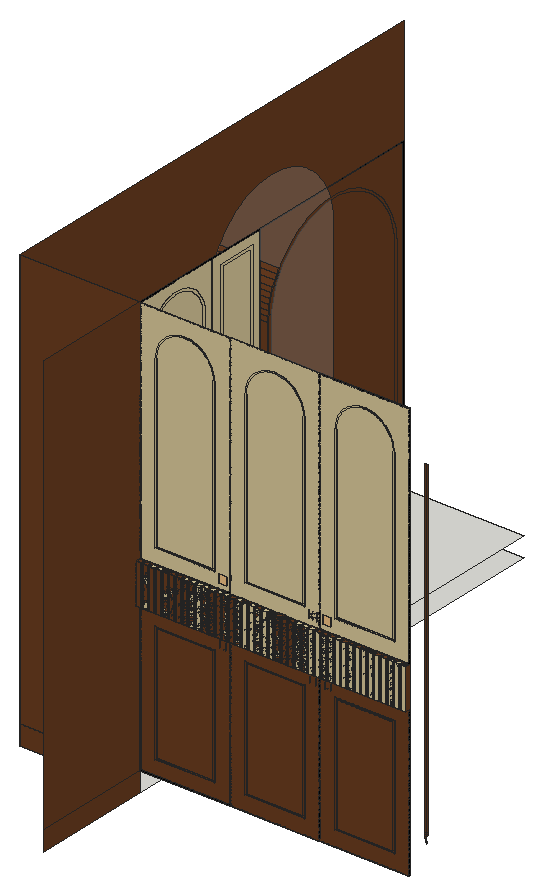
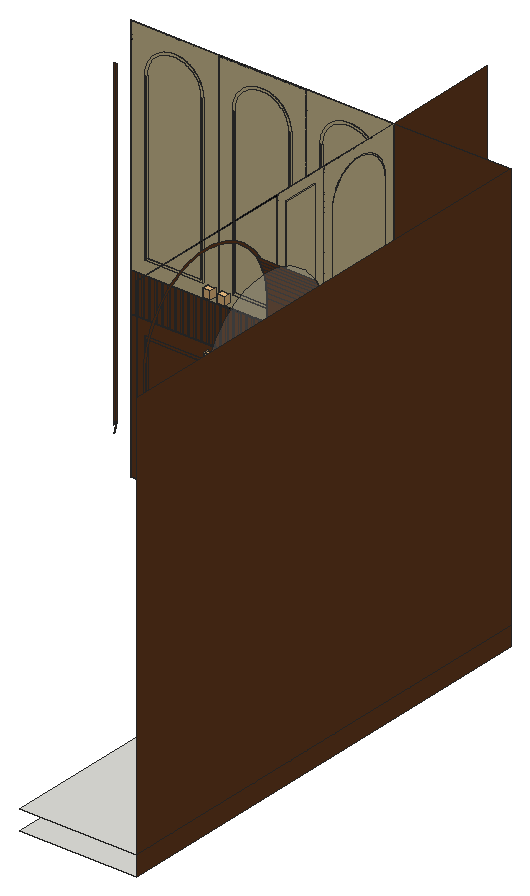
# SketchUp Ruby script. Lengths in inches.
U = 1.inch
M = Sketchup.active_model
def pt(a) = Geom::Point3d.new(a.map { |v| v * U })
def face(e, loops, mat)
  f = e.add_face(loops[0].map { |a| pt(a) })
  loops[1..].each { |l| e.add_face(l.map { |a| pt(a) }).erase! }
  f.material = f.back_material = mat if mat
  f
end
# faces: each face lists its corners as indices into pts; further lists are holes
def faces(e, pts, list, mat = nil) = list.each { |f| face(e, (f[0].is_a?(Array) ? f : [f]).map { |l| l.map { |i| pts[i] } }, mat) }
# xy, xz, yz: faces in a plane at the given z, y or x. An outline is a flat list of corners, or four numbers for a rectangle; further outlines are holes
def ring(l) = l.size == 4 ? [[l[0], l[1]], [l[2], l[1]], [l[2], l[3]], [l[0], l[3]]] : l.each_slice(2).to_a
def flat(e, list, mat, &to3) = list.each { |f| face(e, (f[0].is_a?(Array) ? f : [f]).map { |l| ring(l).map { |u, v| to3.(u, v) } }, mat) }
def xy(e, z, list, mat = nil) = flat(e, list, mat) { |x, y| [x, y, z] }
def xz(e, y, list, mat = nil) = flat(e, list, mat) { |x, z| [x, y, z] }
def yz(e, x, list, mat = nil) = flat(e, list, mat) { |y, z| [x, y, z] }
def lines(e, pts, list) = list.each { |a, b| e.add_line(pt(pts[a]), pt(pts[b])) }
# prism: a flat outline (further loops are holes) pulled along v
def prism(e, loops, v, mat = nil)
  f = face(e, loops, mat); d = Geom::Vector3d.new(v.map { |x| x * U })
  f.pushpull(f.normal.samedirection?(d) ? d.length : -d.length)
end
def box(e, o, s, mat = nil) = prism(e, [[o, [o[0] + s[0], o[1], o[2]], [o[0] + s[0], o[1] + s[1], o[2]], [o[0], o[1] + s[1], o[2]]]], [0, 0, s[2]], mat)
def at(x, y, z, deg = 0) = Geom::Transformation.translation(pt([x, y, z])) * Geom::Transformation.rotation(ORIGIN, Z_AXIS, deg.degrees)
def axes(o, x, y, z) = Geom::Transformation.new([*x, 0, *y, 0, *z, 0, *pt(o).to_a, 1])
def part(name) = M.definitions.add(name)
# library, detail: a bought-in or finely detailed component or shape, given as its bounding box
def library(name, o, s) = part(name).tap { |d| box(d.entities, o, s) }
def detail(e, o, s) = box(e.add_group.entities, o, s)
def put(e, d, t, mat = nil) = e.add_instance(d, t).tap { |i| i.material = mat if mat }
def group(e, t, mat = nil) = e.add_group.tap { |g| g.transformation = t; g.material = mat if mat }.entities
root = M.entities
M.materials.add("138_plaster painted wall texture-seamless").color = [214, 198, 153]
M.materials.add("[0137_Black]").color = [0, 0, 0]
M.materials.add("[Mirror 02]").color = [229, 229, 229]
M.materials["[Mirror 02]"].alpha = 0.23
M.materials.add("[Wood Veneer 01]").color = [104, 60, 32]
c1 = part("Group\#7")
box(c1.entities,[0,0,0],[1,1,8])
c2 = library("Group\#17",[0,0,0],[1.625,1.625,1.31])
xy(root,0,[[0,24,24,120]])
xy(root,4,[[0,24,24,120]])
xy(root,6,[[24,26,24.2,40],[24,44,24.2,52]],"[Wood Veneer 01]")
xy(root,6.4,[[24,26.4,24.2,39.6],[24,44.4,24.2,51.6]],"[Wood Veneer 01]")
xy(root,7,[[27,24,39,24.2]],"138_plaster painted wall texture-seamless")
xy(root,7,[[45,24,57,24.2],[63,24,75,24.2]],"[Wood Veneer 01]")
xy(root,7.4,[[27.4,24,38.6,24.2],[45.4,24,56.6,24.2],[63.4,24,74.6,24.2]],"[Wood Veneer 01]")
xy(root,30.6,[[27.4,24,38.6,24.2]],"138_plaster painted wall texture-seamless")
xy(root,30.6,[[45.4,24,56.6,24.2],[63.4,24,74.6,24.2]],"[Wood Veneer 01]")
xy(root,31,[[27,24,39,24.2],[45,24,57,24.2],[63,24,75,24.2]],"[Wood Veneer 01]")
xy(root,31.6,[[24,26.4,24.2,39.6]])
xy(root,31.6,[[24,44.4,24.2,51.6]],"[Wood Veneer 01]")
xy(root,32,[[24,26,24.2,40],[24,44,24.2,52]],"[Wood Veneer 01]")
xy(root,34,[[24,23,42,24],[42,23,60,24],[60,23,78,24]],"138_plaster painted wall texture-seamless")
xy(root,34,[[23,24,24,42],[23,42,24,54]],"[Wood Veneer 01]")
xy(root,36.4,[[12,56.4,24.2,87.6]],"[Wood Veneer 01]")
xy(root,42,[[24,23,42,24],[42,23,60,24],[60,23,78,24]],"138_plaster painted wall texture-seamless")
xy(root,42,[[23,24,24,42],[23,42,24,54]],"[Wood Veneer 01]")
xy(root,44,[[24,26,24.2,40],[24,44,24.2,52]])
xy(root,44.4,[[24,26.4,24.2,39.6],[24,44.4,24.2,51.6]])
xy(root,45,[[27,24,39,24.2],[45,24,57,24.2],[63,24,75,24.2]],"138_plaster painted wall texture-seamless")
xy(root,45.4,[[27.4,24,38.6,24.2],[45.4,24,56.6,24.2],[63.4,24,74.6,24.2]],"138_plaster painted wall texture-seamless")
xz(root,23,[[24,34,78,42]],"138_plaster painted wall texture-seamless")
xz(root,24,[[[24.1,42.1,41.9,87.9],[27,45,39,45,39,79,38.99,79.35,38.96,79.7,38.91,80.04,38.84,80.38,38.75,80.72,38.64,81.05,38.51,81.375,38.36,81.69,38.2,82,38.01,82.3,37.8125,82.58,37.6,82.86,37.36,83.12,37.12,83.36,36.86,83.6,36.58,83.8125,36.3,84.01,36,84.2,35.69,84.36,35.375,84.51,35.05,84.64,34.72,84.75,34.38,84.84,34.04,84.91,33.7,84.96,33.35,84.99,33,85,32.65,84.99,32.3,84.96,31.96,84.91,31.62,84.84,31.28,84.75,30.95,84.64,30.625,84.51,30.31,84.36,30,84.2,29.7,84.01,29.42,83.8125,29.14,83.6,28.88,83.36,28.64,83.12,28.4,82.86,28.1875,82.58,27.99,82.3,27.8,82,27.64,81.69,27.49,81.375,27.36,81.05,27.25,80.72,27.16,80.38,27.09,80.04,27.04,79.7,27.01,79.35,27,79]],[[42.1,42.1,59.9,87.9],[45,45,57,45,57,79,56.99,79.35,56.96,79.7,56.91,80.04,56.84,80.38,56.75,80.72,56.64,81.05,56.51,81.375,56.36,81.69,56.2,82,56.01,82.3,55.8125,82.58,55.6,82.86,55.36,83.12,55.12,83.36,54.86,83.6,54.58,83.8125,54.3,84.01,54,84.2,53.69,84.36,53.375,84.51,53.05,84.64,52.72,84.75,52.38,84.84,52.04,84.91,51.7,84.96,51.35,84.99,51,85,50.65,84.99,50.3,84.96,49.96,84.91,49.62,84.84,49.28,84.75,48.95,84.64,48.625,84.51,48.31,84.36,48,84.2,47.7,84.01,47.42,83.8125,47.14,83.6,46.88,83.36,46.64,83.12,46.4,82.86,46.1875,82.58,45.99,82.3,45.8,82,45.64,81.69,45.49,81.375,45.36,81.05,45.25,80.72,45.16,80.38,45.09,80.04,45.04,79.7,45.01,79.35,45,79]],[[60.1,42.1,77.9,87.9],[63,45,75,45,75,79,74.99,79.35,74.96,79.7,74.91,80.04,74.84,80.38,74.75,80.72,74.64,81.05,74.51,81.375,74.36,81.69,74.2,82,74.01,82.3,73.8125,82.58,73.6,82.86,73.36,83.12,73.12,83.36,72.86,83.6,72.58,83.8125,72.3,84.01,72,84.2,71.69,84.36,71.375,84.51,71.05,84.64,70.72,84.75,70.38,84.84,70.04,84.91,69.7,84.96,69.35,84.99,69,85,68.65,84.99,68.3,84.96,67.96,84.91,67.62,84.84,67.28,84.75,66.95,84.64,66.625,84.51,66.31,84.36,66,84.2,65.7,84.01,65.42,83.8125,65.14,83.6,64.88,83.36,64.64,83.12,64.4,82.86,64.1875,82.58,63.99,82.3,63.8,82,63.64,81.69,63.49,81.375,63.36,81.05,63.25,80.72,63.16,80.38,63.09,80.04,63.04,79.7,63.01,79.35,63,79]],[27.4,45.4,27.4,79,27.41,79.33,27.4375,79.65,27.49,79.97,27.55,80.29,27.64,80.61,27.74,80.92,27.86,81.22,28,81.51,28.15,81.8,28.32,82.08,28.51,82.34,28.71,82.6,28.93,82.84,29.16,83.07,29.4,83.29,29.66,83.49,29.92,83.68,30.2,83.85,30.49,84,30.78,84.14,31.08,84.26,31.39,84.36,31.71,84.45,32.03,84.51,32.35,84.5625,32.67,84.59,33,84.6,33.33,84.59,33.65,84.5625,33.97,84.51,34.29,84.45,34.61,84.36,34.92,84.26,35.22,84.14,35.51,84,35.8,83.85,36.08,83.68,36.34,83.49,36.6,83.29,36.84,83.07,37.07,82.84,37.29,82.6,37.49,82.34,37.68,82.08,37.85,81.8,38,81.51,38.14,81.22,38.26,80.92,38.36,80.61,38.45,80.29,38.51,79.97,38.5625,79.65,38.59,79.33,38.6,79,38.6,45.4],[45.4,45.4,45.4,79,45.41,79.33,45.4375,79.65,45.49,79.97,45.55,80.29,45.64,80.61,45.74,80.92,45.86,81.22,46,81.51,46.15,81.8,46.32,82.08,46.51,82.34,46.71,82.6,46.93,82.84,47.16,83.07,47.4,83.29,47.66,83.49,47.92,83.68,48.2,83.85,48.49,84,48.78,84.14,49.08,84.26,49.39,84.36,49.71,84.45,50.03,84.51,50.35,84.5625,50.67,84.59,51,84.6,51.33,84.59,51.65,84.5625,51.97,84.51,52.29,84.45,52.61,84.36,52.92,84.26,53.22,84.14,53.51,84,53.8,83.85,54.08,83.68,54.34,83.49,54.6,83.29,54.84,83.07,55.07,82.84,55.29,82.6,55.49,82.34,55.68,82.08,55.85,81.8,56,81.51,56.14,81.22,56.26,80.92,56.36,80.61,56.45,80.29,56.51,79.97,56.5625,79.65,56.59,79.33,56.6,79,56.6,45.4],
  [63.4,45.4,63.4,79,63.41,79.33,63.4375,79.65,63.49,79.97,63.55,80.29,63.64,80.61,63.74,80.92,63.86,81.22,64,81.51,64.15,81.8,64.32,82.08,64.51,82.34,64.71,82.6,64.93,82.84,65.16,83.07,65.4,83.29,65.66,83.49,65.92,83.68,66.2,83.85,66.49,84,66.78,84.14,67.08,84.26,67.39,84.36,67.71,84.45,68.03,84.51,68.35,84.5625,68.67,84.59,69,84.6,69.33,84.59,69.65,84.5625,69.97,84.51,70.29,84.45,70.61,84.36,70.92,84.26,71.22,84.14,71.51,84,71.8,83.85,72.08,83.68,72.34,83.49,72.6,83.29,72.84,83.07,73.07,82.84,73.29,82.6,73.49,82.34,73.68,82.08,73.85,81.8,74,81.51,74.14,81.22,74.26,80.92,74.36,80.61,74.45,80.29,74.51,79.97,74.5625,79.65,74.59,79.33,74.6,79,74.6,45.4]],"138_plaster painted wall texture-seamless")
xz(root,24,[[[24,4,42,34],[24.1,4.1,41.9,33.9]],[[42,4,60,34],[42.1,4.1,59.9,33.9]],[[60,4,78,34],[60.1,4.1,77.9,33.9]],[[24,42,42,88],[24.1,42.1,41.9,87.9]],[[42,42,60,88],[42.1,42.1,59.9,87.9]],
  [[60,42,78,88],[60.1,42.1,77.9,87.9]]],"[0137_Black]")
xz(root,24,[[0,0,24,4],[0,4,24,4,24,34,23,34,23,42,24,42,24,88,0,88],[[24.1,4.1,41.9,33.9],[27,7,39,31]],[[42.1,4.1,59.9,33.9],[45,7,57,31]],[[60.1,4.1,77.9,33.9],[63,7,75,31]],
  [27.4,7.4,38.6,30.6],[45.4,7.4,56.6,30.6],[63.4,7.4,74.6,30.6]],"[Wood Veneer 01]")
xz(root,24.2,[[[27,45,27,79,27.01,79.35,27.04,79.7,27.09,80.04,27.16,80.38,27.25,80.72,27.36,81.05,27.49,81.375,27.64,81.69,27.8,82,27.99,82.3,28.1875,82.58,28.4,82.86,28.64,83.12,28.88,83.36,29.14,83.6,29.42,83.8125,29.7,84.01,30,84.2,30.31,84.36,30.625,84.51,30.95,84.64,31.28,84.75,31.62,84.84,31.96,84.91,32.3,84.96,32.65,84.99,33,85,33.35,84.99,33.7,84.96,34.04,84.91,34.38,84.84,34.72,84.75,35.05,84.64,35.375,84.51,35.69,84.36,36,84.2,36.3,84.01,36.58,83.8125,36.86,83.6,37.12,83.36,37.36,83.12,37.6,82.86,37.8125,82.58,38.01,82.3,38.2,82,38.36,81.69,38.51,81.375,38.64,81.05,38.75,80.72,38.84,80.38,38.91,80.04,38.96,79.7,38.99,79.35,39,79,39,45],[27.4,45.4,38.6,45.4,38.6,79,38.59,79.33,38.5625,79.65,38.51,79.97,38.45,80.29,38.36,80.61,38.26,80.92,38.14,81.22,38,81.51,37.85,81.8,37.68,82.08,37.49,82.34,37.29,82.6,37.07,82.84,36.84,83.07,36.6,83.29,36.34,83.49,36.08,83.68,35.8,83.85,35.51,84,35.22,84.14,34.92,84.26,34.61,84.36,34.29,84.45,33.97,84.51,33.65,84.5625,33.33,84.59,33,84.6,32.67,84.59,32.35,84.5625,32.03,84.51,31.71,84.45,31.39,84.36,31.08,84.26,30.78,84.14,30.49,84,30.2,83.85,29.92,83.68,29.66,83.49,29.4,83.29,29.16,83.07,28.93,82.84,28.71,82.6,28.51,82.34,28.32,82.08,28.15,81.8,28,81.51,27.86,81.22,27.74,80.92,27.64,80.61,27.55,80.29,27.49,79.97,27.4375,79.65,27.41,79.33,27.4,79]],[[45,45,45,79,45.01,79.35,45.04,79.7,45.09,80.04,45.16,80.38,45.25,80.72,45.36,81.05,45.49,81.375,45.64,81.69,45.8,82,45.99,82.3,46.1875,82.58,46.4,82.86,46.64,83.12,46.88,83.36,47.14,83.6,47.42,83.8125,47.7,84.01,48,84.2,48.31,84.36,48.625,84.51,48.95,84.64,49.28,84.75,49.62,84.84,49.96,84.91,50.3,84.96,50.65,84.99,51,85,51.35,84.99,51.7,84.96,52.04,84.91,52.38,84.84,52.72,84.75,53.05,84.64,53.375,84.51,53.69,84.36,54,84.2,54.3,84.01,54.58,83.8125,54.86,83.6,55.12,83.36,55.36,83.12,55.6,82.86,55.8125,82.58,56.01,82.3,56.2,82,56.36,81.69,56.51,81.375,56.64,81.05,56.75,80.72,56.84,80.38,56.91,80.04,56.96,79.7,56.99,79.35,57,79,57,45],[45.4,45.4,56.6,45.4,56.6,79,56.59,79.33,56.5625,79.65,56.51,79.97,56.45,80.29,56.36,80.61,56.26,80.92,56.14,81.22,56,81.51,55.85,81.8,55.68,82.08,55.49,82.34,55.29,82.6,55.07,82.84,54.84,83.07,54.6,83.29,54.34,83.49,54.08,83.68,53.8,83.85,53.51,84,53.22,84.14,52.92,84.26,52.61,84.36,52.29,84.45,51.97,84.51,51.65,84.5625,51.33,84.59,51,84.6,50.67,84.59,50.35,84.5625,50.03,84.51,49.71,84.45,49.39,84.36,49.08,84.26,48.78,84.14,48.49,84,48.2,83.85,47.92,83.68,47.66,83.49,47.4,83.29,47.16,83.07,46.93,82.84,46.71,82.6,46.51,82.34,46.32,82.08,46.15,81.8,46,81.51,45.86,81.22,45.74,80.92,45.64,80.61,45.55,80.29,45.49,79.97,45.4375,79.65,45.41,79.33,45.4,79]],[[63,45,63,79,63.01,79.35,63.04,79.7,63.09,80.04,63.16,80.38,63.25,80.72,63.36,81.05,63.49,81.375,63.64,81.69,63.8,82,63.99,82.3,64.1875,82.58,64.4,82.86,64.64,83.12,64.88,83.36,65.14,83.6,65.42,83.8125,65.7,84.01,66,84.2,66.31,84.36,66.625,84.51,66.95,84.64,67.28,84.75,67.62,84.84,67.96,84.91,68.3,84.96,68.65,84.99,69,85,69.35,84.99,69.7,84.96,70.04,84.91,70.38,84.84,70.72,84.75,71.05,84.64,71.375,84.51,71.69,84.36,72,84.2,72.3,84.01,72.58,83.8125,72.86,83.6,73.12,83.36,73.36,83.12,73.6,82.86,73.8125,82.58,74.01,82.3,74.2,82,74.36,81.69,74.51,81.375,74.64,81.05,74.75,80.72,74.84,80.38,74.91,80.04,74.96,79.7,74.99,79.35,75,79,75,45],[63.4,45.4,74.6,45.4,74.6,79,74.59,79.33,74.5625,79.65,74.51,79.97,74.45,80.29,74.36,80.61,74.26,80.92,74.14,81.22,74,81.51,73.85,81.8,73.68,82.08,73.49,82.34,73.29,82.6,73.07,82.84,72.84,83.07,72.6,83.29,72.34,83.49,72.08,83.68,71.8,83.85,71.51,84,71.22,84.14,70.92,84.26,70.61,84.36,70.29,84.45,69.97,84.51,69.65,84.5625,69.33,84.59,69,84.6,68.67,84.59,68.35,84.5625,68.03,84.51,67.71,84.45,67.39,84.36,67.08,84.26,66.78,84.14,66.49,84,66.2,83.85,65.92,83.68,65.66,83.49,65.4,83.29,65.16,83.07,64.93,82.84,64.71,82.6,64.51,82.34,64.32,82.08,64.15,81.8,64,81.51,63.86,81.22,63.74,80.92,63.64,80.61,63.55,80.29,63.49,79.97,63.4375,79.65,63.41,79.33,63.4,79]]],"138_plaster painted wall texture-seamless")
xz(root,24.2,[[[27,7,39,31],[27.4,7.4,38.6,30.6]],[[45,7,57,31],[45.4,7.4,56.6,30.6]],[[63,7,75,31],[63.4,7.4,74.6,30.6]]],"[Wood Veneer 01]")
xz(root,26,[[24,6,24.2,32],[24,44,24.2,79]])
xz(root,26.4,[[24,44.4,24.2,79]])
xz(root,26.4,[[24,6.4,24.2,31.6]],"[Wood Veneer 01]")
xz(root,39.6,[[24,44.4,24.2,79]])
xz(root,39.6,[[24,6.4,24.2,31.6]],"[Wood Veneer 01]")
xz(root,40,[[24,44,24.2,79]])
xz(root,40,[[24,6,24.2,32]],"[Wood Veneer 01]")
xz(root,44,[[24,44,24.2,86]])
xz(root,44,[[24,6,24.2,32]],"[Wood Veneer 01]")
xz(root,44.4,[[24,44.4,24.2,85.6]])
xz(root,44.4,[[24,6.4,24.2,31.6]],"[Wood Veneer 01]")
xz(root,51.6,[[24,44.4,24.2,85.6]])
xz(root,51.6,[[24,6.4,24.2,31.6]],"[Wood Veneer 01]")
xz(root,52,[[24,44,24.2,86]])
xz(root,52,[[24,6,24.2,32]],"[Wood Veneer 01]")
xz(root,54,[[23,34,24,42]])
xz(root,56,[[24,6,24.2,12],[24,16,24.2,22],[24,26,24.2,32],[24,36,24.2,42],[24,42,24.2,70]],"[Wood Veneer 01]")
xz(root,56.4,[[24,6.4,24.2,11.6],[24,16.4,24.2,21.6],[24,26.4,24.2,31.6],[12,36.4,24.2,70]],"[Wood Veneer 01]")
yz(root,0,[[24,0,120,4],[24,4,120,88]],"[Wood Veneer 01]")
yz(root,12,[[56.4,36.4,87.6,36.4,87.6,70,87.57,71.02,87.47,72.04,87.3,73.04,87.07,74.04,86.77,75.01,86.41,75.97,85.99,76.9,85.51,77.8,84.97,78.67,84.375,79.5,83.73,80.29,83.03,81.03,82.29,81.73,81.5,82.375,80.67,82.97,79.8,83.51,78.9,83.99,77.97,84.41,77.01,84.77,76.04,85.07,75.04,85.3,74.04,85.47,73.02,85.57,72,85.6,70.98,85.57,69.96,85.47,68.96,85.3,67.96,85.07,66.99,84.77,66.03,84.41,65.1,83.99,64.2,83.51,63.33,82.97,62.5,82.375,61.71,81.73,60.97,81.03,60.27,80.29,59.625,79.5,59.03,78.67,58.49,77.8,58.01,76.9,57.59,75.97,57.23,75.01,56.93,74.04,56.7,73.04,56.53,72.04,56.43,71.02,56.4,70]],"[Mirror 02]")
yz(root,23,[[24,34,54,42]],"[Wood Veneer 01]")
yz(root,24,[[[24.1,42.1,41.9,87.9],[26,44,26,79,26.01,79.46,26.06,79.91,26.13,80.37,26.24,80.8125,26.37,81.25,26.53,81.68,26.72,82.1,26.9375,82.5,27.18,82.89,27.45,83.26,27.74,83.62,28.05,83.95,28.38,84.26,28.74,84.55,29.11,84.82,29.5,85.0625,29.9,85.28,30.32,85.47,30.75,85.63,31.1875,85.76,31.63,85.87,32.09,85.94,32.54,85.99,33,86,33.46,85.99,33.91,85.94,34.37,85.87,34.8125,85.76,35.25,85.63,35.68,85.47,36.1,85.28,36.5,85.0625,36.89,84.82,37.26,84.55,37.62,84.26,37.95,83.95,38.26,83.62,38.55,83.26,38.82,82.89,39.0625,82.5,39.28,82.1,39.47,81.68,39.63,81.25,39.76,80.8125,39.87,80.37,39.94,79.91,39.99,79.46,40,79,40,44]],[[42.1,42.1,53.9,87.9],[44,44,52,86]],[26.4,44.4,39.6,44.4,39.6,79,39.59,79.43,39.54,79.86,39.47,80.29,39.375,80.71,39.25,81.12,39.1,81.53,38.92,81.92,38.72,82.3,38.49,82.67,38.24,83.02,37.96,83.35,37.67,83.67,37.35,83.96,37.02,84.24,36.67,84.49,36.3,84.72,35.92,84.92,35.53,85.1,35.12,85.25,34.71,85.375,34.29,85.47,33.86,85.54,33.43,85.59,33,85.6,32.57,85.59,32.14,85.54,31.71,85.47,31.29,85.375,30.88,85.25,30.47,85.1,30.08,84.92,29.7,84.72,29.33,84.49,28.98,84.24,28.65,83.96,28.33,83.67,28.04,83.35,27.76,83.02,27.51,82.67,27.28,82.3,27.08,81.92,26.9,81.53,26.75,81.12,26.625,80.71,26.53,80.29,26.46,79.86,26.41,79.43,26.4,79],[44.4,44.4,51.6,85.6]],"138_plaster painted wall texture-seamless")
yz(root,24,[[[24,4,42,34],[24.1,4.1,41.9,33.9]],[[42,4,54,34],[42.1,4.1,53.9,33.9]],[[54,4,90,14],[54.1,4.1,89.9,13.9]],[[54,14,90,24],[54.1,14.1,89.9,23.9]],[[54,24,90,34],[54.1,24.1,89.9,33.9]],
  [[54,34,90,88],[54.1,34.1,89.9,87.9]],[[24,42,42,88],[24.1,42.1,41.9,87.9]],[[42,42,54,88],[42.1,42.1,53.9,87.9]]],"[0137_Black]")
yz(root,24,[[0,0,24,4],[0,4,0,88,24,88,24,42,23,42,23,34,24,34,24,4],[[24.1,4.1,41.9,33.9],[26,6,40,32]],[[42.1,4.1,53.9,33.9],[44,6,52,32]],[[54.1,4.1,89.9,13.9],[56,6,88,12]],
  [26.4,6.4,39.6,31.6],[44.4,6.4,51.6,31.6],[56.4,6.4,87.6,11.6],[[54.1,14.1,89.9,23.9],[56,16,88,22]],[56.4,16.4,87.6,21.6],
  [[54.1,24.1,89.9,33.9],[56,26,88,32]],[56.4,26.4,87.6,31.6]],"[Wood Veneer 01]")
yz(root,24.2,[[[26,44,40,44,40,79,39.99,79.46,39.94,79.91,39.87,80.37,39.76,80.8125,39.63,81.25,39.47,81.68,39.28,82.1,39.0625,82.5,38.82,82.89,38.55,83.26,38.26,83.62,37.95,83.95,37.62,84.26,37.26,84.55,36.89,84.82,36.5,85.0625,36.1,85.28,35.68,85.47,35.25,85.63,34.8125,85.76,34.37,85.87,33.91,85.94,33.46,85.99,33,86,32.54,85.99,32.09,85.94,31.63,85.87,31.1875,85.76,30.75,85.63,30.32,85.47,29.9,85.28,29.5,85.0625,29.11,84.82,28.74,84.55,28.38,84.26,28.05,83.95,27.74,83.62,27.45,83.26,27.18,82.89,26.9375,82.5,26.72,82.1,26.53,81.68,26.37,81.25,26.24,80.8125,26.13,80.37,26.06,79.91,26.01,79.46,26,79],[26.4,44.4,26.4,79,26.41,79.43,26.46,79.86,26.53,80.29,26.625,80.71,26.75,81.12,26.9,81.53,27.08,81.92,27.28,82.3,27.51,82.67,27.76,83.02,28.04,83.35,28.33,83.67,28.65,83.96,28.98,84.24,29.33,84.49,29.7,84.72,30.08,84.92,30.47,85.1,30.88,85.25,31.29,85.375,31.71,85.47,32.14,85.54,32.57,85.59,33,85.6,33.43,85.59,33.86,85.54,34.29,85.47,34.71,85.375,35.12,85.25,35.53,85.1,35.92,84.92,36.3,84.72,36.67,84.49,37.02,84.24,37.35,83.96,37.67,83.67,37.96,83.35,38.24,83.02,38.49,82.67,38.72,82.3,38.92,81.92,39.1,81.53,39.25,81.12,39.375,80.71,39.47,80.29,39.54,79.86,39.59,79.43,39.6,79,39.6,44.4]],[[44,44,52,86],[44.4,44.4,51.6,85.6]]],"138_plaster painted wall texture-seamless")
yz(root,24.2,[[[26,6,40,32],[26.4,6.4,39.6,31.6]],[[44,6,52,32],[44.4,6.4,51.6,31.6]],[[56,36,88,36,88,70,87.97,71.05,87.86,72.09,87.69,73.12,87.45,74.14,87.15,75.14,86.78,76.12,86.35,77.08,85.86,78,85.3,78.89,84.69,79.74,84.03,80.55,83.3125,81.3125,82.55,82.03,81.74,82.69,80.89,83.3,80,83.86,79.08,84.35,78.12,84.78,77.14,85.15,76.14,85.45,75.12,85.69,74.09,85.86,73.05,85.97,72,86,70.95,85.97,69.91,85.86,68.88,85.69,67.86,85.45,66.86,85.15,65.88,84.78,64.92,84.35,64,83.86,63.11,83.3,62.26,82.69,61.45,82.03,60.6875,81.3125,59.97,80.55,59.31,79.74,58.7,78.89,58.14,78,57.65,77.08,57.22,76.12,56.85,75.14,56.55,74.14,56.31,73.12,56.14,72.09,56.03,71.05,56,70],[56.4,36.4,56.4,70,56.43,71.02,56.53,72.04,56.7,73.04,56.93,74.04,57.23,75.01,57.59,75.97,58.01,76.9,58.49,77.8,59.03,78.67,59.625,79.5,60.27,80.29,60.97,81.03,61.71,81.73,62.5,82.375,63.33,82.97,64.2,83.51,65.1,83.99,66.03,84.41,66.99,84.77,67.96,85.07,68.96,85.3,69.96,85.47,70.98,85.57,72,85.6,73.02,85.57,74.04,85.47,75.04,85.3,76.04,85.07,77.01,84.77,77.97,84.41,78.9,83.99,79.8,83.51,80.67,82.97,81.5,82.375,82.29,81.73,83.03,81.03,83.73,80.29,84.375,79.5,84.97,78.67,85.51,77.8,85.99,76.9,86.41,75.97,86.77,75.01,87.07,74.04,87.3,73.04,87.47,72.04,87.57,71.02,87.6,70,87.6,36.4]]],"[Wood Veneer 01]")
yz(root,27,[[24,45,24.2,79]],"138_plaster painted wall texture-seamless")
yz(root,27,[[24,7,24.2,31]],"[Wood Veneer 01]")
yz(root,27.4,[[24,45.4,24.2,79]],"138_plaster painted wall texture-seamless")
yz(root,27.4,[[24,7.4,24.2,30.6]],"[Wood Veneer 01]")
yz(root,38.6,[[24,45.4,24.2,79]],"138_plaster painted wall texture-seamless")
yz(root,38.6,[[24,7.4,24.2,30.6]],"[Wood Veneer 01]")
yz(root,39,[[24,45,24.2,79]],"138_plaster painted wall texture-seamless")
yz(root,39,[[24,7,24.2,31]],"[Wood Veneer 01]")
yz(root,45,[[24,45,24.2,79]],"138_plaster painted wall texture-seamless")
yz(root,45,[[24,7,24.2,31]],"[Wood Veneer 01]")
yz(root,45.4,[[24,45.4,24.2,79]],"138_plaster painted wall texture-seamless")
yz(root,45.4,[[24,7.4,24.2,30.6]],"[Wood Veneer 01]")
yz(root,56.6,[[24,45.4,24.2,79]],"138_plaster painted wall texture-seamless")
yz(root,56.6,[[24,7.4,24.2,30.6]],"[Wood Veneer 01]")
yz(root,57,[[24,45,24.2,79]],"138_plaster painted wall texture-seamless")
yz(root,57,[[24,7,24.2,31]],"[Wood Veneer 01]")
yz(root,63,[[24,45,24.2,79]],"138_plaster painted wall texture-seamless")
yz(root,63,[[24,7,24.2,31]],"[Wood Veneer 01]")
yz(root,63.4,[[24,45.4,24.2,79]],"138_plaster painted wall texture-seamless")
yz(root,63.4,[[24,7.4,24.2,30.6]],"[Wood Veneer 01]")
yz(root,74.6,[[24,45.4,24.2,79]],"138_plaster painted wall texture-seamless")
yz(root,74.6,[[24,7.4,24.2,30.6]],"[Wood Veneer 01]")
yz(root,75,[[24,45,24.2,79]],"138_plaster painted wall texture-seamless")
yz(root,75,[[24,7,24.2,31]],"[Wood Veneer 01]")
yz(root,78,[[23,34,24,42]],"138_plaster painted wall texture-seamless")
yz(root,81,[[24,13,24.2,79]],"[Wood Veneer 01]")
yz(root,81.4,[[24,13,24.2,79]],"[Wood Veneer 01]")
p = [[81.36,24,10.95],[81.25,24,11.28],[81.25,24.2,11.28],[81.36,24.2,10.95],[81.16,24,11.62],[81.16,24.2,11.62],
  [81.09,24,11.96],[81.09,24.2,11.96],[81.04,24,12.3],[81.04,24.2,12.3],[81.01,24,12.65],[81.01,24.2,12.65],
  [81.41,24,12.67],[81.4375,24,12.35],[81.4375,24.2,12.35],[81.41,24.2,12.67],[81,24,13],[81,24.2,13],
  [81.4,24,13],[81.4,24.2,13],[24,56.03,71.05],[24,56,70],[24.2,56,70],[24.2,56.03,71.05],
  [12,56.43,71.02],[24.2,56.43,71.02],[24.2,56.4,70],[12,56.4,70],[24,56.14,72.09],[24.2,56.14,72.09],
  [12,56.53,72.04],[24.2,56.53,72.04],[12,56.7,73.04],[24.2,56.7,73.04],[24,56.31,73.12],[24.2,56.31,73.12],
  [12,56.93,74.04],[24.2,56.93,74.04],[24,56.55,74.14],[24.2,56.55,74.14],[12,57.23,75.01],[24.2,57.23,75.01],
  [24,56.85,75.14],[24.2,56.85,75.14],[12,57.59,75.97],[24.2,57.59,75.97],[24,57.22,76.12],[24.2,57.22,76.12],
  [12,58.01,76.9],[24.2,58.01,76.9],[24,57.65,77.08],[24.2,57.65,77.08],[12,58.49,77.8],[24.2,58.49,77.8],
  [24,58.14,78],[24.2,58.14,78],[12,59.03,78.67],[24.2,59.03,78.67],[24,58.7,78.89],[24.2,58.7,78.89]]
faces(root,p,[[0,1,2,3],[1,4,5,2],[4,6,7,5],[6,8,9,7],[8,10,11,9],[12,13,14,15],[10,16,17,11],[18,12,15,19],
  [20,21,22,23],[24,25,26,27],[28,20,23,29],[30,31,25,24],[32,33,31,30],[34,28,29,35],[36,37,33,32],[38,34,35,39],
  [40,41,37,36],[42,38,39,43],[44,45,41,40],[46,42,43,47],[48,49,45,44],[50,46,47,51],[52,53,49,48],[54,50,51,55],
  [56,57,53,52],[58,54,55,59]],"[Wood Veneer 01]")
g1 = group(root,at(24,23,34),"[Wood Veneer 01]")
put(g1,c1,at(42.4,0,0))
put(g1,c1,at(37.1,0,0))
put(g1,c1,at(33.125,0,0))
put(g1,c1,at(7.95,0,0))
put(g1,c1,at(38.43,0,0))
put(g1,c1,at(35.78,0,0))
put(g1,c1,at(50.35,0,0))
put(g1,c1,at(49.03,0,0))
put(g1,c1,at(43.73,0,0))
put(g1,c1,at(47.7,0,0))
put(g1,c1,at(39.75,0,0))
put(g1,c1,at(45.05,0,0))
put(g1,c1,at(46.375,0,0))
put(g1,c1,at(41.08,0,0))
put(g1,c1,at(31.8,0,0))
put(g1,c1,at(34.45,0,0))
put(g1,c1,at(51.68,0,0))
put(g1,c1,at(30.48,0,0))
put(g1,c1,at(27.83,0,0))
put(g1,c1,at(9.28,0,0))
put(g1,c1,at(14.58,0,0))
put(g1,c1,at(13.25,0,0))
put(g1,c1,at(18.55,0,0))
put(g1,c1,at(17.23,0,0))
put(g1,c1,at(10.6,0,0))
put(g1,c1,at(22.53,0,0))
put(g1,c1,at(23.85,0,0))
put(g1,c1,at(26.5,0,0))
put(g1,c1,at(21.2,0,0))
put(g1,c1,at(15.9,0,0))
put(g1,c1,at(25.18,0,0))
put(g1,c1,at(11.93,0,0))
put(g1,c1,at(19.875,0,0))
put(g1,c1,at(53,0,0))
put(g1,c1,at(29.15,0,0))
put(g1,c1,at(2.65,0,0))
put(g1,c1,at(3.97,0,0))
put(g1,c1,at(6.625,0,0))
put(g1,c1,at(5.3,0,0))
put(g1,c1,at(1.32,0,0))
put(g1,c1,at(0,0,0))
put(root,c2,axes([40.06,24,32.84],[0.75,0,0],[0,0,-0.75],[0,0.75,0]),"[Wood Veneer 01]")
put(root,c2,axes([58.06,24,32.84],[0.75,0,0],[0,0,-0.75],[0,0.75,0]),"[Wood Veneer 01]")
put(root,c2,axes([60.93,24,32.84],[0.75,0,0],[0,0,-0.75],[0,0.75,0]),"[Wood Veneer 01]")
put(root,c1,at(23,24,34),"[Wood Veneer 01]")
put(root,c2,axes([39.72,24,44.81],[1,0,0],[0,0,-1],[0,1,0]),"[Wood Veneer 01]")
put(root,c2,axes([57.72,24,44.81],[1,0,0],[0,0,-1],[0,1,0]),"[Wood Veneer 01]")
put(root,c2,axes([60.66,24,44.81],[1,0,0],[0,0,-1],[0,1,0]),"[Wood Veneer 01]")
put(root,c1,at(23,25.26,34),"[Wood Veneer 01]")
put(root,c1,at(23,26.52,34),"[Wood Veneer 01]")
put(root,c1,at(23,27.78,34),"[Wood Veneer 01]")
put(root,c1,at(23,29.04,34),"[Wood Veneer 01]")
put(root,c1,at(23,30.3,34),"[Wood Veneer 01]")
put(root,c1,at(23,31.57,34),"[Wood Veneer 01]")
put(root,c1,at(23,32.83,34),"[Wood Veneer 01]")
put(root,c1,at(23,34.09,34),"[Wood Veneer 01]")
put(root,c1,at(23,35.35,34),"[Wood Veneer 01]")
put(root,c1,at(23,36.61,34),"[Wood Veneer 01]")
put(root,c1,at(23,37.87,34),"[Wood Veneer 01]")
put(root,c1,at(23,39.13,34),"[Wood Veneer 01]")
put(root,c1,at(23,40.39,34),"[Wood Veneer 01]")
put(root,c2,axes([24,41.5625,43.94],[0,-0.74,0],[0,0,-0.74],[0.74,0,0]),"[Wood Veneer 01]")
put(root,c2,axes([24,41.57,33.29],[0,-0.74,0],[0,0,-0.74],[0.74,0,0]),"[Wood Veneer 01]")
put(root,c1,at(23,41.65,34),"[Wood Veneer 01]")
put(root,c2,axes([24,43.6875,43.94],[0,-0.74,0],[0,0,-0.74],[0.74,0,0]),"[Wood Veneer 01]")
put(root,c2,axes([24,43.82,33.29],[0,-0.74,0],[0,0,-0.74],[0.74,0,0]),"[Wood Veneer 01]")
put(root,c1,at(23,42.91,34),"[Wood Veneer 01]")
put(root,c1,at(23,44.17,34),"[Wood Veneer 01]")
put(root,c1,at(23,45.43,34),"[Wood Veneer 01]")
put(root,c1,at(23,46.7,34),"[Wood Veneer 01]")
put(root,c1,at(23,47.96,34),"[Wood Veneer 01]")
put(root,c1,at(23,49.22,34),"[Wood Veneer 01]")
put(root,c1,at(23,50.48,34),"[Wood Veneer 01]")
put(root,c1,at(23,51.74,34),"[Wood Veneer 01]")
put(root,c1,at(23,53,34),"[Wood Veneer 01]")
put(root,c2,axes([24,72.45,9.77],[0,-0.74,0],[0,0,-0.74],[0.74,0,0]),"[Wood Veneer 01]")
put(root,c2,axes([24,72.45,19.77],[0,-0.74,0],[0,0,-0.74],[0.74,0,0]),"[Wood Veneer 01]")
put(root,c2,axes([24,72.45,29.77],[0,-0.74,0],[0,0,-0.74],[0.74,0,0]),"[Wood Veneer 01]")
